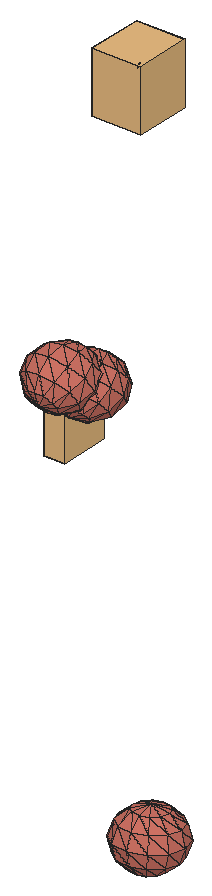
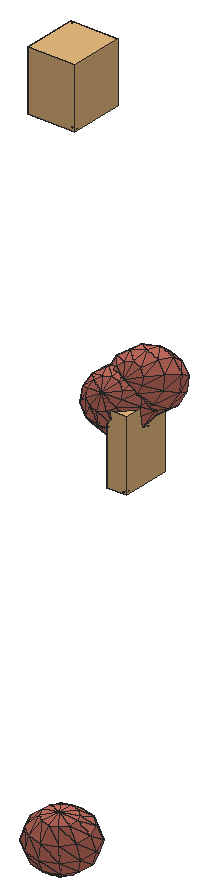
# SketchUp Ruby script. Lengths in inches.
U = 1.inch
M = Sketchup.active_model
def pt(a) = Geom::Point3d.new(a.map { |v| v * U })
def face(e, loops, mat)
  f = e.add_face(loops[0].map { |a| pt(a) })
  loops[1..].each { |l| e.add_face(l.map { |a| pt(a) }).erase! }
  f.material = f.back_material = mat if mat
  f
end
# faces: each face lists its corners as indices into pts; further lists are holes
def faces(e, pts, list, mat = nil) = list.each { |f| face(e, (f[0].is_a?(Array) ? f : [f]).map { |l| l.map { |i| pts[i] } }, mat) }
# xy, xz, yz: faces in a plane at the given z, y or x. An outline is a flat list of corners, or four numbers for a rectangle; further outlines are holes
def ring(l) = l.size == 4 ? [[l[0], l[1]], [l[2], l[1]], [l[2], l[3]], [l[0], l[3]]] : l.each_slice(2).to_a
def flat(e, list, mat, &to3) = list.each { |f| face(e, (f[0].is_a?(Array) ? f : [f]).map { |l| ring(l).map { |u, v| to3.(u, v) } }, mat) }
def xy(e, z, list, mat = nil) = flat(e, list, mat) { |x, y| [x, y, z] }
def xz(e, y, list, mat = nil) = flat(e, list, mat) { |x, z| [x, y, z] }
def yz(e, x, list, mat = nil) = flat(e, list, mat) { |y, z| [x, y, z] }
def lines(e, pts, list) = list.each { |a, b| e.add_line(pt(pts[a]), pt(pts[b])) }
# prism: a flat outline (further loops are holes) pulled along v
def prism(e, loops, v, mat = nil)
  f = face(e, loops, mat); d = Geom::Vector3d.new(v.map { |x| x * U })
  f.pushpull(f.normal.samedirection?(d) ? d.length : -d.length)
end
def box(e, o, s, mat = nil) = prism(e, [[o, [o[0] + s[0], o[1], o[2]], [o[0] + s[0], o[1] + s[1], o[2]], [o[0], o[1] + s[1], o[2]]]], [0, 0, s[2]], mat)
def at(x, y, z, deg = 0) = Geom::Transformation.translation(pt([x, y, z])) * Geom::Transformation.rotation(ORIGIN, Z_AXIS, deg.degrees)
def axes(o, x, y, z) = Geom::Transformation.new([*x, 0, *y, 0, *z, 0, *pt(o).to_a, 1])
def part(name) = M.definitions.add(name)
# library, detail: a bought-in or finely detailed component or shape, given as its bounding box
def library(name, o, s) = part(name).tap { |d| box(d.entities, o, s) }
def detail(e, o, s) = box(e.add_group.entities, o, s)
def put(e, d, t, mat = nil) = e.add_instance(d, t).tap { |i| i.material = mat if mat }
def group(e, t, mat = nil) = e.add_group.tap { |g| g.transformation = t; g.material = mat if mat }.entities
root = M.entities
M.materials.add("green").color = [174, 139, 102]
M.materials.add("vio").color = [206, 114, 100]
c1 = part("3DGeom~194_Defintion")
p = [[111.52,-262.8,-376.52],[-124.92,-186.52,-431.46],[-6.51,0,-500],[214.07,-101.27,-435.87],[-225.34,101.27,-430.15],[113.66,186.52,-434.56],
  [-121.28,262.8,-373.49],[318.08,-268.67,-220.68],[318.08,-268.67,-220.68],[377.29,-175.41,-254.95],[377.29,-175.41,-254.95],[318.13,60.26,-379.2],
  [318.13,60.26,-379.2],[318.13,60.26,-379.2],[203.36,323.0625,-252.6875],[-43.59,381.05,-215.98],[-43.59,381.05,-215.98],[203.36,323.0625,-252.6875],
  [37.95,-381.05,-217.04],[-209.87,-323.0625,-247.3125],[37.95,-381.05,-217.04],[-327.89,-60.26,-370.8],[-327.89,-60.26,-370.8],[-383.79,175.41,-245.05],
  [-225.34,101.27,-430.15],[-383.79,175.41,-245.05],[-323.71,268.67,-212.33],[-323.71,268.67,-212.33],[377.29,-175.41,-254.95],[318.13,60.26,-379.2],
  [437.37,-82.15,-222.23],[437.37,-82.15,-222.23],[318.13,60.26,-379.2],[395.82,178.51,-221.69],[318.13,60.26,-379.2],[203.36,323.0625,-252.6875],
  [395.82,178.51,-221.69],[275.6,-336.9375,-128.61],[37.95,-381.05,-217.04],[111.52,-262.8,-376.52],[275.6,-336.9375,-128.61],[111.52,-262.8,-376.52],
  [318.08,-268.67,-220.68],[-121.28,262.8,-373.49],[-323.71,268.67,-212.33],[-278.86,336.9375,-121.39],[-121.28,262.8,-373.49],[-43.59,381.05,-215.98],
  [-401.46,-178.51,-211.32],[-401.46,-178.51,-211.32],[-443,82.15,-210.78],[-327.89,-60.26,-370.8],[-327.89,-60.26,-370.8],[-383.79,175.41,-245.05],
  [318.08,-268.67,-220.68],[377.29,-175.41,-254.95],[439.41,-202.54,-5.72],[203.36,323.0625,-252.6875],[238.58,373.04,-3.1],[203.36,323.0625,-252.6875],
  [-13.09,424.33,0.17],[203.36,323.0625,-252.6875],[238.58,373.04,-3.1],[13.09,-424.33,-0.17],[-238.58,-373.04,3.1],[-209.87,-323.0625,-247.3125],
  [-209.87,-323.0625,-247.3125],[-238.58,-373.04,3.1],[-401.46,-178.51,-211.32],[-209.87,-323.0625,-247.3125],[-383.79,175.41,-245.05],[-439.41,202.54,5.72],
  [-323.71,268.67,-212.33],[-383.79,175.41,-245.05],[482.22,-13.88,-131.3],[426.32,221.79,-5.55],[275.6,-336.9375,-128.61],[261.25,-361.93,-3.4],
  [261.25,-361.93,-3.4],[275.6,-336.9375,-128.61],[-261.25,361.93,3.4],[-278.86,336.9375,-121.39],[-323.71,268.67,-212.33],[-238.58,-373.04,3.1],
  [-426.32,-221.79,5.55],[-401.46,-178.51,-211.32],[-485.47,13.88,-118.7],[-401.46,-178.51,-211.32],[-401.46,-178.51,-211.32],[499.83,11.11,-6.5],
  [261.25,-361.93,-3.4],[-261.25,361.93,3.4],[-278.86,336.9375,-121.39],[-499.83,-11.11,6.5],[485.47,-13.88,118.7],[401.46,178.51,211.32],
  [278.86,-336.9375,121.39],[323.71,-268.67,212.33],[383.79,-175.41,245.05],[443,-82.15,210.78],[209.87,323.0625,247.3125],[209.87,323.0625,247.3125],
  [278.86,-336.9375,121.39],[261.25,-361.93,-3.4],[238.58,373.04,-3.1],[-37.95,381.05,217.04],[209.87,323.0625,247.3125],[238.58,373.04,-3.1],
  [-37.95,381.05,217.04],[43.59,-381.05,215.98],[278.86,-336.9375,121.39],[-275.6,336.9375,128.61],[-37.95,381.05,217.04],[-203.36,-323.0625,252.6875],
  [-203.36,-323.0625,252.6875],[-238.58,-373.04,3.1],[-275.6,336.9375,128.61],[-261.25,361.93,3.4],[-203.36,-323.0625,252.6875],[-395.82,-178.51,221.69],
  [-482.22,13.88,131.3],[-437.37,82.15,222.23],[-377.29,175.41,254.95],[-377.29,175.41,254.95],[-318.08,268.67,220.68],[-318.08,268.67,220.68],
  [-275.6,336.9375,128.61],[327.89,60.26,370.8],[323.71,-268.67,212.33],[278.86,-336.9375,121.39],[-37.95,381.05,217.04],[-318.08,268.67,220.68],
  [-318.13,-60.26,379.2],[-318.13,-60.26,379.2],[225.34,-101.27,430.15],[225.34,-101.27,430.15],[401.46,178.51,211.32],[124.92,186.52,431.46],
  [327.89,60.26,370.8],[401.46,178.51,211.32],[209.87,323.0625,247.3125],[323.71,-268.67,212.33],[121.28,-262.8,373.49],[383.79,-175.41,245.05],
  [121.28,-262.8,373.49],[323.71,-268.67,212.33],[121.28,-262.8,373.49],[-203.36,-323.0625,252.6875],[43.59,-381.05,215.98],[-37.95,381.05,217.04],
  [-318.08,268.67,220.68],[-111.52,262.8,376.51],[-37.95,381.05,217.04],[-111.52,262.8,376.51],[-318.08,268.67,220.68],[-377.29,175.41,254.95],
  [-113.66,-186.52,434.56],[-395.82,-178.51,221.69],[-203.36,-323.0625,252.6875],[-318.13,-60.26,379.2],[-395.82,-178.51,221.69],[-214.07,101.27,435.87],
  [-437.37,82.15,222.23],[-437.37,82.15,222.23],[383.79,-175.41,245.05],[225.34,-101.27,430.15],[121.28,-262.8,373.49],[121.28,-262.8,373.49],
  [-203.36,-323.0625,252.6875],[327.89,60.26,370.8],[6.51,0,500],[327.89,60.26,370.8],[121.28,-262.8,373.49]]
faces(c1.entities,p,[[0,1,2],[0,2,3],[1,4,2],[3,2,5],[2,4,6],[2,6,5],[7,0,3],[8,3,9],
  [10,3,11],[3,5,12],[13,5,14],[5,6,15],[5,16,17],[18,19,1],[20,1,0],[19,21,1],
  [1,21,4],[22,23,24],[4,25,26],[4,27,6],[28,29,30],[31,32,33],[34,35,36],[37,38,39],
  [40,41,42],[43,44,45],[46,45,47],[19,48,21],[49,50,51],[52,50,53],[54,55,56],[55,31,56],
  [33,57,58],[59,47,60],[61,60,62],[63,64,65],[63,66,38],[67,68,69],[70,50,71],[72,73,71],
  [31,74,56],[31,33,74],[74,33,75],[33,58,75],[76,54,56],[77,63,38],[78,38,79],[47,45,80],
  [47,80,60],[81,82,71],[83,84,85],[84,86,87],[88,86,50],[50,86,71],[74,89,56],[74,75,89],
  [90,76,56],[91,92,71],[84,93,86],[86,93,71],[89,94,56],[89,95,94],[89,75,95],[96,90,56],
  [97,96,56],[98,97,56],[99,98,56],[94,99,56],[75,100,95],[75,58,101],[102,63,103],[104,105,106],
  [107,60,108],[109,64,63],[110,109,63],[60,80,111],[60,111,112],[109,113,64],[114,84,115],[116,117,71],
  [118,119,84],[119,93,84],[93,120,71],[120,121,71],[121,122,71],[123,124,71],[125,126,71],[119,120,93],
  [94,127,99],[94,95,127],[128,109,129],[130,111,131],[132,120,119],[133,121,120],[99,134,98],[99,127,135],
  [136,137,138],[139,140,137],[141,142,109],[143,144,145],[146,147,148],[149,150,151],[140,152,153],[153,154,155],
  [156,157,158],[156,159,160],[161,162,159],[161,155,163],[164,165,166],[140,153,137],[167,156,168],[153,155,161],
  [169,170,165],[171,137,170],[165,156,172],[137,153,161],[170,159,156],[170,161,159],[165,170,156],[137,161,170]],"vio")
c2 = part("3DGeom~224_Defintion")
p = [[81.72,-275.8,-371.94],[-133.11,-167.42,-440.41],[24.02,0,-500],[217.8,-130.81,-423.55],[-176.2,130.81,-442.48],[217.8,-130.81,-423.55],
  [174.72,167.42,-425.62],[-45.69,275.8,-378.0625],[-312.28,-14.1875,-390.87],[-329.21,226.5625,-266.39],[-253.86,310.28,-229.2],[-253.86,310.28,-229.2],
  [-23.47,-381.94,-218.13],[-254.58,-289.99,-262.81],[-23.47,-381.94,-218.13],[217.8,-130.81,-423.55],[348.3125,14.1875,-359.13],[348.3125,14.1875,-359.13],
  [278.6,289.99,-237.19],[44.27,381.94,-214.88],[44.27,381.94,-214.88],[278.6,289.99,-237.19],[274.66,-310.28,-203.8125],[217.8,-130.81,-423.55],
  [274.66,-310.28,-203.8125],[217.8,-130.81,-423.55],[353.23,-226.5625,-233.61],[353.23,-226.5625,-233.61],[217.8,-130.81,-423.55],[348.3125,14.1875,-359.13],
  [-417.47,-120.33,-237.0625],[-417.47,-120.33,-237.0625],[-407.77,142.85,-236.59],[-312.28,-14.1875,-390.87],[-407.77,142.85,-236.59],[-45.69,275.8,-378.0625],
  [-253.86,310.28,-229.2],[-201.92,371.56,-134.99],[-45.69,275.8,-378.0625],[44.27,381.94,-214.88],[213.93,-371.56,-115.01],[-23.47,-381.94,-218.13],
  [81.72,-275.8,-371.94],[213.93,-371.56,-115.01],[81.72,-275.8,-371.94],[274.66,-310.28,-203.8125],[428.58,-142.85,-196.42],[438.28,120.33,-195.95],
  [348.3125,14.1875,-359.13],[278.6,289.99,-237.19],[438.28,120.33,-195.95],[-329.21,226.5625,-266.39],[-407.77,142.85,-236.59],[-394.01,261.61,-18.93],
  [-253.86,310.28,-229.2],[-329.21,226.5625,-266.39],[-69.59,-420.79,-3.34],[-307.83,-334.85,-14.79],[-254.58,-289.99,-262.81],[-254.58,-289.99,-262.81],
  [-307.83,-334.85,-14.79],[-417.47,-120.33,-237.0625],[-254.58,-289.99,-262.81],[278.6,289.99,-237.19],[307.83,334.85,14.79],[278.6,289.99,-237.19],
  [69.59,420.79,3.34],[278.6,289.99,-237.19],[307.83,334.85,14.79],[-307.83,-334.85,-14.79],[-463.59,-159.18,-22.27],[-417.47,-120.33,-237.0625],
  [-468.51,81.57,-147.8],[-417.47,-120.33,-237.0625],[-417.47,-120.33,-237.0625],[-407.77,142.85,-236.59],[-407.77,142.85,-236.59],[274.66,-310.28,-203.8125],
  [394.01,-261.61,18.93],[394.01,-261.61,18.93],[-201.92,371.56,-134.99],[-253.86,310.28,-229.2],[187.3,-393.99,9],[213.93,-371.56,-115.01],
  [-187.3,393.99,-9],[213.93,-371.56,-115.01],[394.01,-261.61,18.93],[480.52,-81.57,-102.2],[394.01,-261.61,18.93],[463.59,159.18,22.27],
  [-495.13,59.14,-23.79],[-394.01,261.61,-18.93],[213.93,-371.56,-115.01],[394.01,-261.61,18.93],[495.13,-59.14,23.79],[394.01,-261.61,18.93],
  [-438.28,-120.33,195.95],[-480.52,81.57,102.2],[-278.6,-289.99,237.19],[-307.83,-334.85,-14.79],[-278.6,-289.99,237.19],[-428.58,142.85,196.42],
  [-353.23,226.5625,233.61],[-274.66,310.28,203.8125],[-274.66,310.28,203.8125],[-213.93,371.56,115.01],[-213.93,371.56,115.01],[-394.01,261.61,-18.93],
  [-44.27,-381.94,214.88],[-278.6,-289.99,237.19],[201.92,-371.56,134.99],[307.83,334.85,14.79],[23.47,381.94,218.13],[23.47,381.94,218.13],
  [254.58,289.99,262.81],[307.83,334.85,14.79],[23.47,381.94,218.13],[254.58,289.99,262.81],[253.86,-310.28,229.2],[201.92,-371.56,134.99],
  [394.01,-261.61,18.93],[329.21,-226.5625,266.39],[394.01,-261.61,18.93],[407.77,-142.85,236.59],[394.01,-261.61,18.93],[468.51,-81.57,147.8],
  [394.01,-261.61,18.93],[394.01,-261.61,18.93],[417.47,120.33,237.0625],[254.58,289.99,262.81],[-348.3125,-14.1875,359.13],[-348.3125,-14.1875,359.13],
  [23.47,381.94,218.13],[-274.66,310.28,203.8125],[253.86,-310.28,229.2],[312.28,14.1875,390.87],[312.28,14.1875,390.87],[-174.72,-167.42,425.62],
  [-438.28,-120.33,195.95],[-278.6,-289.99,237.19],[-348.3125,-14.1875,359.13],[-438.28,-120.33,195.95],[-217.8,130.81,423.55],[-348.3125,-14.1875,359.13],
  [-217.8,130.81,423.55],[-81.72,275.8,371.94],[-274.66,310.28,203.8125],[-353.23,226.5625,233.61],[23.47,381.94,218.13],[-274.66,310.28,203.8125],
  [-81.72,275.8,371.94],[45.69,-275.8,378.0625],[-278.6,-289.99,237.19],[-44.27,-381.94,214.88],[253.86,-310.28,229.2],[45.69,-275.8,378.0625],
  [254.58,289.99,262.81],[23.47,381.94,218.13],[329.21,-226.5625,266.39],[45.69,-275.8,378.0625],[253.86,-310.28,229.2],[-353.23,226.5625,233.61],
  [-217.8,130.81,423.55],[407.77,-142.85,236.59],[176.2,-130.81,442.48],[329.21,-226.5625,266.39],[407.77,-142.85,236.59],[312.28,14.1875,390.87],
  [417.47,120.33,237.0625],[133.11,167.42,440.41],[417.47,120.33,237.0625],[45.69,-275.8,378.0625],[-278.6,-289.99,237.19],[329.21,-226.5625,266.39],
  [45.69,-275.8,378.0625],[-24.02,0,500],[45.69,-275.8,378.0625]]
faces(c2.entities,p,[[0,1,2],[0,2,3],[1,4,2],[5,2,6],[2,4,7],[2,7,6],[1,8,4],[8,9,4],
  [4,9,10],[4,11,7],[12,13,1],[14,1,0],[13,8,1],[15,6,16],[17,6,18],[6,7,19],
  [6,20,21],[22,0,23],[24,25,26],[27,28,29],[13,30,8],[31,32,33],[8,34,9],[35,36,37],
  [38,37,39],[40,41,42],[43,44,45],[27,29,46],[46,29,47],[48,49,50],[51,52,53],[54,55,53],
  [56,57,58],[56,59,41],[60,61,62],[47,63,64],[65,39,66],[67,66,68],[69,70,71],[70,72,73],
  [74,72,75],[76,72,53],[77,27,78],[27,46,79],[80,81,53],[82,56,41],[82,41,83],[39,37,84],
  [39,84,66],[85,77,86],[46,87,88],[46,47,87],[87,47,89],[47,64,89],[70,90,72],[72,90,53],
  [84,37,91],[82,92,93],[87,94,95],[87,89,94],[96,90,70],[96,97,90],[90,97,53],[98,70,99],
  [100,96,70],[97,101,53],[101,102,53],[102,103,53],[104,105,53],[106,84,107],[108,57,56],[108,109,57],
  [66,84,106],[110,108,56],[110,56,82],[111,66,112],[66,106,113],[110,82,93],[89,64,114],[115,116,117],
  [118,119,120],[121,118,122],[123,121,124],[125,123,126],[94,125,127],[94,89,128],[89,129,128],[94,128,125],
  [130,97,96],[131,101,97],[132,106,133],[134,108,110],[125,135,123],[125,128,136],[137,138,139],[137,140,141],
  [142,101,143],[144,102,101],[145,146,147],[148,149,150],[151,152,153],[154,155,108],[156,157,145],[158,159,160],
  [145,161,162],[163,164,165],[166,167,164],[168,169,167],[170,156,169],[171,137,172],[156,145,169],[173,164,174],
  [175,140,137],[175,162,140],[169,145,162],[164,137,176],[167,175,164],[167,169,175],[169,162,175],[164,175,137]],"vio")
c3 = library("3DGeom~19_Defintion",[-341.38,-500,-142.11],[682.76,1000,284.22])
c4 = part("3DGeom~20_Defintion")
p = [[-311.06,-487.18,-72.26],[-310.25,-484.5,-142.11],[-284.25,-498.77,-90.07],[-284.25,-498.77,-90.07],[-310.25,-484.5,-142.11],[-283.85,-497.43,-124.99],
  [-310.25,-484.5,-142.11],[-294.95,-491.76,-137.63],[-283.85,-497.43,-124.99],[-337.46,-474.24,-89.375],[-310.25,-484.5,-142.11],[-311.06,-487.18,-72.26],
  [-337.0625,-472.9,-124.3],[-310.25,-484.5,-142.11],[-337.46,-474.24,-89.375],[-310.25,-484.5,-142.11],[-337.0625,-472.9,-124.3],[-325.67,-477.6,-137.23],
  [-284.25,-498.77,-90.07],[-283.85,-497.43,-124.99],[-279.93,-500,-107.58],[-337.0625,-472.9,-124.3],[-337.46,-474.24,-89.375],[-341.38,-471.67,-106.78],
  [-311.06,-487.18,-72.26],[-284.25,-498.77,-90.07],[-295.64,-494.08,-77.14],[-337.46,-474.24,-89.375],[-311.06,-487.18,-72.26],[-326.37,-479.92,-76.74],
  [319.0625,494.74,82.9],[301.91,466.72,142.11],[318.42,461.52,137.94],[319.0625,494.74,82.9],[318.42,461.52,137.94],[332.8,461.46,126.96],
  [319.0625,494.74,82.9],[332.8,461.46,126.96],[341.21,466.57,112.1],[319.0625,494.74,82.9],[341.21,466.57,112.1],[341.38,475.47,97.35],
  [319.0625,494.74,82.9],[287.69,475.68,138.34],[301.91,466.72,142.11],[319.0625,494.74,82.9],[341.38,475.47,97.35],[333.27,485.79,86.67],
  [319.0625,494.74,82.9],[279.59,485.99,127.65],[287.69,475.68,138.34],[319.0625,494.74,82.9],[279.76,494.89,112.9],[279.59,485.99,127.65],
  [319.0625,494.74,82.9],[288.17,500,98.05],[279.76,494.89,112.9],[319.0625,494.74,82.9],[302.55,499.95,87.06],[288.17,500,98.05]]
faces(c4.entities,p,[[0,1,2],[3,4,5],[6,7,8],[9,10,11],[12,13,14],[15,16,17],[18,19,20],[21,22,23],
  [24,25,26],[27,28,29],[30,31,32],[33,34,35],[36,37,38],[39,40,41],[42,43,44],[45,46,47],
  [48,49,50],[51,52,53],[54,55,56],[57,58,59]],"green")
c5 = library("3DGeom~9_Defintion",[-447.05,-500,-392.82],[894.1,1000,785.64])
c6 = part("3DGeom~10_Defintion")
p = [[-376.65,-477.04,-383.86],[-408.2,-455.37,-392.67],[-389.75,-464.73,-392.82],[-376.65,-477.04,-383.86],[-442.82,-474.42,-333.72],[-408.2,-455.37,-392.67],
  [-408.2,-455.37,-392.67],[-442.82,-474.42,-333.72],[-441.29,-454.05,-367.6],[-408.2,-455.37,-392.67],[-441.29,-454.05,-367.6],[-427.07,-451.46,-383.43],
  [-378.18,-497.41,-349.98],[-442.82,-474.42,-333.72],[-376.65,-477.04,-383.86],[-378.18,-497.41,-349.98],[-376.65,-477.04,-383.86],[-372.41,-489,-368.18],
  [-442.82,-474.42,-333.72],[-447.05,-462.46,-349.4],[-441.29,-454.05,-367.6],[-411.26,-496.09,-324.91],[-378.18,-497.41,-349.98],[-392.4,-500,-334.15],
  [-411.26,-496.09,-324.91],[-442.82,-474.42,-333.72],[-378.18,-497.41,-349.98],[-442.82,-474.42,-333.72],[-411.26,-496.09,-324.91],[-429.72,-486.73,-324.76],
  [401.4,485.85,384.88],[441.04,458.37,319.44],[429.72,472.35,311.5],[401.4,485.85,384.88],[429.72,472.35,311.5],[416.12,486.26,314.46],
  [401.4,485.85,384.88],[416.12,486.26,314.46],[403.89,496.38,327.52],[401.4,485.85,384.88],[447.05,448.07,336.15],[441.04,458.37,319.44],
  [401.4,485.85,384.88],[403.89,496.38,327.52],[396.3,500,347.18],[401.4,485.85,384.88],[446.15,444.22,357.14],[447.05,448.07,336.15],
  [401.4,485.85,384.88],[396.3,500,347.18],[395.39,496.14,368.18],[401.4,485.85,384.88],[438.56,447.84,376.81],[446.15,444.22,357.14],
  [401.4,485.85,384.88],[426.33,457.96,389.87],[438.56,447.84,376.81],[401.4,485.85,384.88],[412.73,471.87,392.82],[426.33,457.96,389.87]]
faces(c6.entities,p,[[0,1,2],[3,4,5],[6,7,8],[9,10,11],[12,13,14],[15,16,17],[18,19,20],[21,22,23],
  [24,25,26],[27,28,29],[30,31,32],[33,34,35],[36,37,38],[39,40,41],[42,43,44],[45,46,47],
  [48,49,50],[51,52,53],[54,55,56],[57,58,59]],"green")
c7 = part("3DGeom~192_Defintion")
p = [[46.59,-12.33,-500],[-151.08,-242.85,-384.34],[-208.06,-36.06,-455.29],[69.45,-222.31,-423.06],[288.76,14.69,-410.73],[11.25,200.94,-442.97],
  [220.97,224.35,-365.66],[-323.33,-255.02,-239.97],[-406.96,-50.11,-288.59],[-323.33,-255.02,-239.97],[-209.29,180.4,-404.25],[-406.96,-50.11,-288.59],
  [-27.11,360.38,-267.25],[93.97,373.89,-222.61],[-27.11,360.38,-267.25],[93.97,373.89,-222.61],[-53.62,-384.57,-210.4],[73.7,-372.71,-232.75],
  [-53.62,-384.57,-210.4],[279.17,-198.9,-345.75],[453.55,37.78,-211.41],[279.17,-198.9,-345.75],[288.76,14.69,-410.73],[363.68,244.34,-193.04],
  [288.76,14.69,-410.73],[220.97,224.35,-365.66],[363.68,244.34,-193.04],[288.76,14.69,-410.73],[-406.96,-50.11,-288.59],[-381.54,168.23,-259.88],
  [-154.4375,348.52,-244.89],[-381.54,168.23,-259.88],[-27.11,360.38,-267.25],[-154.4375,348.52,-244.89],[-151.08,-242.85,-384.34],[-153.07,-391.6,-127.05],
  [-323.33,-255.02,-239.97],[-151.08,-242.85,-384.34],[-53.62,-384.57,-210.4],[176.37,385.43,-122.95],[220.97,224.35,-365.66],[93.97,373.89,-222.61],
  [363.68,244.34,-193.04],[220.97,224.35,-365.66],[194.79,-359.2,-188.12],[421.89,-178.91,-173.13],[194.79,-359.2,-188.12],[279.17,-198.9,-345.75],
  [279.17,-198.9,-345.75],[-406.96,-50.11,-288.59],[-401.15,-255.57,-28.63],[-496.8125,-50.74,-44.56],[-323.33,-255.02,-239.97],[-381.54,168.23,-259.88],
  [-27.11,360.38,-267.25],[-154.4375,348.52,-244.89],[-58.21,423.25,-19.91],[-459.36,167.68,-48.54],[-253.89,341.49,-161.54],[-154.4375,348.52,-244.89],
  [-381.54,168.23,-259.88],[-253.89,341.49,-161.54],[-253.89,341.49,-161.54],[-323.33,-255.02,-239.97],[-198,-391.92,-5.03],[-401.15,-255.57,-28.63],
  [-323.33,-255.02,-239.97],[73.7,-372.71,-232.75],[58.21,-423.25,19.91],[73.7,-372.71,-232.75],[194.79,-359.2,-188.12],[496.8125,50.74,44.56],
  [401.15,255.57,28.63],[363.68,244.34,-193.04],[401.15,255.57,28.63],[198,391.92,5.03],[401.15,255.57,28.63],[194.79,-359.2,-188.12],
  [277.18,-347.66,-88.46],[277.18,-347.66,-88.46],[194.79,-359.2,-188.12],[459.36,-167.68,48.55],[-253.89,341.49,-161.54],[-298.81,341.17,-39.53],
  [-298.81,341.17,-39.53],[277.18,-347.66,-88.46],[298.81,-341.17,39.53],[298.81,-341.17,39.53],[-453.55,-37.78,211.41],[-421.89,178.91,173.13],
  [-298.81,341.17,-39.53],[-363.68,-244.34,193.05],[-298.81,341.17,-39.53],[-277.18,347.66,88.46],[-277.18,347.66,88.46],[-401.15,-255.57,-28.63],
  [-176.37,-385.43,122.95],[-401.15,-255.57,-28.63],[-363.68,-244.34,193.05],[-194.79,359.2,188.12],[-73.7,372.71,232.75],[53.62,384.57,210.4],
  [153.07,391.6,127.05],[-93.97,-373.89,222.61],[27.11,-360.38,267.25],[-93.97,-373.89,222.61],[154.4375,-348.52,244.89],[27.11,-360.38,267.25],
  [298.81,-341.17,39.53],[253.89,-341.49,161.54],[253.89,-341.49,161.54],[154.4375,-348.52,244.89],[323.33,255.02,239.97],[401.15,255.57,28.63],
  [323.33,255.02,239.97],[381.54,-168.23,259.88],[253.89,-341.49,161.54],[406.96,50.11,288.59],[323.33,255.02,239.97],[-277.18,347.66,88.46],
  [-279.17,198.9,345.75],[-277.18,347.66,88.46],[-279.17,198.9,345.75],[-194.79,359.2,188.12],[-363.68,-244.34,193.05],[-93.97,-373.89,222.61],
  [209.29,-180.4,404.25],[154.4375,-348.52,244.89],[253.89,-341.49,161.54],[253.89,-341.49,161.54],[381.54,-168.23,259.88],[-288.76,-14.69,410.73],
  [-288.76,-14.69,410.73],[-279.17,198.9,345.75],[-194.79,359.2,188.12],[-279.17,198.9,345.75],[-69.45,222.31,423.06],[-194.79,359.2,188.12],
  [-73.7,372.71,232.75],[-363.68,-244.34,193.05],[-93.97,-373.89,222.61],[-220.97,-224.35,365.66],[-220.97,-224.35,365.66],[-73.7,372.71,232.75],
  [151.08,242.85,384.34],[53.62,384.57,210.4],[151.08,242.85,384.34],[-220.97,-224.35,365.66],[-288.76,-14.69,410.73],[-220.97,-224.35,365.66],
  [-93.97,-373.89,222.61],[27.11,-360.38,267.25],[-73.7,372.71,232.75],[151.08,242.85,384.34],[151.08,242.85,384.34],[406.96,50.11,288.59],
  [323.33,255.02,239.97],[-11.25,-200.94,442.97],[208.06,36.05,455.29],[381.54,-168.23,259.88],[381.54,-168.23,259.88],[406.96,50.11,288.59],
  [151.08,242.85,384.34],[406.96,50.11,288.59],[-288.76,-14.69,410.73],[-46.59,12.33,500],[151.08,242.85,384.34]]
faces(c7.entities,p,[[0,1,2],[0,3,1],[4,3,0],[5,0,2],[6,0,5],[6,4,0],[2,7,8],[2,1,9],
  [10,2,11],[5,2,10],[12,5,10],[13,5,14],[15,6,5],[3,16,1],[3,17,18],[19,17,3],
  [4,19,3],[20,21,22],[23,24,25],[26,20,27],[10,28,29],[30,10,31],[32,10,33],[34,35,36],
  [37,38,35],[39,40,41],[39,42,43],[19,44,17],[45,46,47],[20,45,48],[49,50,51],[49,52,50],
  [53,49,51],[54,55,56],[41,54,56],[53,51,57],[58,53,57],[59,60,61],[55,62,56],[63,64,65],
  [66,35,64],[38,67,68],[69,70,68],[39,41,56],[71,45,20],[72,20,73],[74,71,20],[35,38,68],
  [75,42,39],[75,76,42],[77,78,68],[45,79,80],[81,79,45],[71,81,45],[82,57,83],[62,84,56],
  [64,35,68],[75,39,56],[85,86,68],[81,87,79],[57,51,88],[57,88,89],[90,57,89],[51,50,91],
  [51,91,88],[92,89,93],[84,94,56],[95,64,96],[97,96,98],[94,99,56],[99,100,56],[100,101,56],
  [101,102,56],[102,75,56],[96,64,68],[102,76,75],[103,96,68],[104,105,68],[106,107,68],[108,109,68],
  [110,111,68],[112,71,113],[102,114,76],[115,116,87],[115,87,81],[117,81,71],[118,117,71],[117,115,81],
  [119,89,120],[121,122,123],[124,96,125],[101,114,102],[126,127,128],[126,129,130],[89,88,131],[89,132,133],
  [134,135,136],[137,136,138],[139,140,141],[88,91,142],[143,144,145],[101,146,114],[88,147,148],[149,150,151],
  [152,136,153],[154,155,156],[157,151,127],[157,127,126],[158,126,159],[158,160,161],[149,151,157],[162,158,163],
  [135,164,165],[135,165,136],[164,149,157],[136,158,166],[165,157,126],[165,126,158],[164,157,165],[136,165,158]],"vio")
g1 = group(root,at(15.3125,134.49,26.21))
put(g1,c1,axes([3.29,-0.23,13.07],[0,0.00039,0],[0,0,-0.00039],[-0.00039,0,0]),"vio")
g2 = group(root,at(15.3125,134.49,26.21))
put(g2,c2,axes([3.35,-0.11,13],[0,0.00039,0],[0,0,-0.00039],[-0.00039,0,0]),"vio")
g3 = group(root,at(15.3125,134.49,26.21))
put(g3,c3,axes([3.24,-0.08,12.83],[0,0.00042,0],[0,0,-0.00042],[-0.00042,0,0]),"green")
put(g3,c4,axes([3.24,-0.08,12.83],[0,0.00042,0],[0,0,-0.00042],[-0.00042,0,0]),"green")
g4 = group(root,at(15.3125,134.49,26.21))
put(g4,c5,axes([3.6,-0.06,14.67],[0,0.00036,0],[0,0,-0.00036],[-0.00036,0,0]),"green")
put(g4,c6,axes([3.6,-0.06,14.67],[0,0.00036,0],[0,0,-0.00036],[-0.00036,0,0]),"green")
g5 = group(root,at(15.3125,134.49,26.21))
put(g5,c7,axes([3.57,0.06,10.63],[0,0.00039,0],[0,0,-0.00039],[-0.00039,0,0]),"vio")
